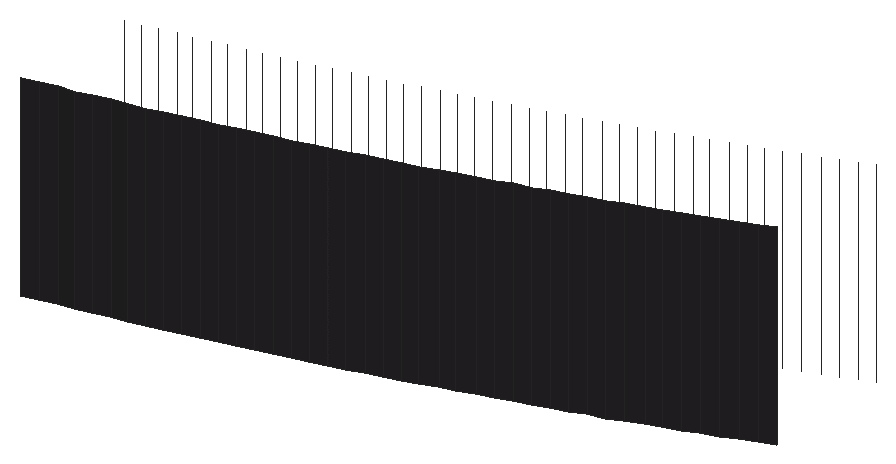
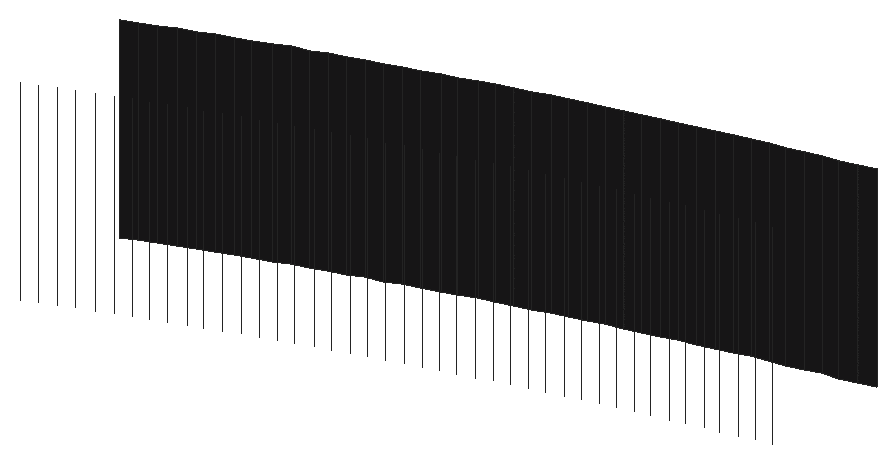
# SketchUp Ruby script. Lengths in inches.
U = 1.inch
M = Sketchup.active_model
def pt(a) = Geom::Point3d.new(a.map { |v| v * U })
def face(e, loops, mat)
  f = e.add_face(loops[0].map { |a| pt(a) })
  loops[1..].each { |l| e.add_face(l.map { |a| pt(a) }).erase! }
  f.material = f.back_material = mat if mat
  f
end
# faces: each face lists its corners as indices into pts; further lists are holes
def faces(e, pts, list, mat = nil) = list.each { |f| face(e, (f[0].is_a?(Array) ? f : [f]).map { |l| l.map { |i| pts[i] } }, mat) }
# xy, xz, yz: faces in a plane at the given z, y or x. An outline is a flat list of corners, or four numbers for a rectangle; further outlines are holes
def ring(l) = l.size == 4 ? [[l[0], l[1]], [l[2], l[1]], [l[2], l[3]], [l[0], l[3]]] : l.each_slice(2).to_a
def flat(e, list, mat, &to3) = list.each { |f| face(e, (f[0].is_a?(Array) ? f : [f]).map { |l| ring(l).map { |u, v| to3.(u, v) } }, mat) }
def xy(e, z, list, mat = nil) = flat(e, list, mat) { |x, y| [x, y, z] }
def xz(e, y, list, mat = nil) = flat(e, list, mat) { |x, z| [x, y, z] }
def yz(e, x, list, mat = nil) = flat(e, list, mat) { |y, z| [x, y, z] }
def lines(e, pts, list) = list.each { |a, b| e.add_line(pt(pts[a]), pt(pts[b])) }
# prism: a flat outline (further loops are holes) pulled along v
def prism(e, loops, v, mat = nil)
  f = face(e, loops, mat); d = Geom::Vector3d.new(v.map { |x| x * U })
  f.pushpull(f.normal.samedirection?(d) ? d.length : -d.length)
end
def box(e, o, s, mat = nil) = prism(e, [[o, [o[0] + s[0], o[1], o[2]], [o[0] + s[0], o[1] + s[1], o[2]], [o[0], o[1] + s[1], o[2]]]], [0, 0, s[2]], mat)
def at(x, y, z, deg = 0) = Geom::Transformation.translation(pt([x, y, z])) * Geom::Transformation.rotation(ORIGIN, Z_AXIS, deg.degrees)
def axes(o, x, y, z) = Geom::Transformation.new([*x, 0, *y, 0, *z, 0, *pt(o).to_a, 1])
def part(name) = M.definitions.add(name)
# library, detail: a bought-in or finely detailed component or shape, given as its bounding box
def library(name, o, s) = part(name).tap { |d| box(d.entities, o, s) }
def detail(e, o, s) = box(e.add_group.entities, o, s)
def put(e, d, t, mat = nil) = e.add_instance(d, t).tap { |i| i.material = mat if mat }
def group(e, t, mat = nil) = e.add_group.tap { |g| g.transformation = t; g.material = mat if mat }.entities
root = M.entities
M.materials.add("Marble_07_1K").color = [36, 34, 36]
p = [[350.16,772.86,18],[350.24,772.88,18],[350.24,772.88,19],[350.16,772.86,19],[350.32,772.9,18],[350.32,772.9,19],
  [350.4,772.91,18],[350.4,772.91,19],[350.47,772.93,18],[350.47,772.93,19],[350.55,772.95,18],[350.55,772.95,19],
  [350.63,772.96,18],[350.63,772.96,19],[350.71,772.98,18],[350.71,772.98,19],[350.78,773,18],[350.78,773,19],
  [350.86,773.02,18],[350.86,773.02,19],[350.9375,773.04,18],[350.9375,773.04,19],[351.02,773.06,18],[351.02,773.06,19],
  [351.09,773.08,18],[351.09,773.08,19],[351.17,773.1,18],[351.17,773.1,19],[351.25,773.12,18],[351.25,773.12,19],
  [351.33,773.14,18],[351.33,773.14,19],[351.4,773.16,18],[351.4,773.16,19],[351.48,773.18,18],[351.48,773.18,19],
  [351.56,773.2,18],[351.56,773.2,19],[351.63,773.23,18],[351.63,773.23,19],[351.71,773.25,18],[351.71,773.25,19],
  [351.79,773.27,18],[351.79,773.27,19],[351.86,773.29,18],[351.86,773.29,19],[351.9375,773.32,18],[351.9375,773.32,19],
  [352.01,773.34,18],[352.01,773.34,19],[352.09,773.37,18],[352.09,773.37,19],[352.17,773.39,18],[352.17,773.39,19],
  [352.24,773.42,18],[352.24,773.42,19],[352.32,773.44,18],[352.32,773.44,19],[352.39,773.47,18],[352.39,773.47,19],
  [352.47,773.49,18],[352.47,773.49,19],[352.54,773.52,18],[352.54,773.52,19],[352.62,773.54,18],[352.62,773.54,19],
  [352.69,773.57,18],[352.69,773.57,19],[352.77,773.6,18],[352.77,773.6,19],[352.84,773.625,18],[352.84,773.625,19],
  [352.92,773.65,18],[352.92,773.65,19],[352.99,773.68,18],[352.99,773.68,19],[353.07,773.71,18],[353.07,773.71,19],
  [353.14,773.74,18],[353.14,773.74,19],[353.22,773.77,18],[353.22,773.77,19],[353.29,773.8,18],[353.29,773.8,19],
  [350.19,773.49,18],[350.19,773.49,19],[350.27,773.5,18],[350.27,773.5,19],[350.34,773.52,18],[350.34,773.52,19],
  [350.42,773.54,18],[350.42,773.54,19],[350.49,773.55,18],[350.49,773.55,19],[350.57,773.57,18],[350.57,773.57,19],
  [350.64,773.59,18],[350.64,773.59,19],[350.72,773.61,18],[350.72,773.61,19],[350.79,773.625,18],[350.79,773.625,19],
  [350.87,773.64,18],[350.87,773.64,19],[350.94,773.66,18],[350.94,773.66,19],[351.02,773.68,18],[351.02,773.68,19],
  [351.09,773.7,18],[351.09,773.7,19],[351.17,773.72,18],[351.17,773.72,19],[351.24,773.74,18],[351.24,773.74,19],
  [351.32,773.76,18],[351.32,773.76,19],[351.39,773.78,18],[351.39,773.78,19],[351.46,773.81,18],[351.46,773.81,19],
  [351.54,773.83,18],[351.54,773.83,19],[351.61,773.85,18],[351.61,773.85,19],[351.68,773.87,18],[351.68,773.87,19],
  [351.76,773.89,18],[351.76,773.89,19],[351.83,773.92,18],[351.83,773.92,19],[351.91,773.94,18],[351.91,773.94,19],
  [351.98,773.96,18],[351.98,773.96,19],[352.05,773.99,18],[352.05,773.99,19],[352.125,774.01,18],[352.125,774.01,19],
  [352.2,774.04,18],[352.2,774.04,19],[352.27,774.0625,18],[352.27,774.0625,19],[352.34,774.09,18],[352.34,774.09,19],
  [352.42,774.11,18],[352.42,774.11,19],[352.49,774.14,18],[352.49,774.14,19],[352.5625,774.17,18],[352.5625,774.17,19],
  [352.63,774.19,18],[352.63,774.19,19],[352.71,774.22,18],[352.71,774.22,19],[352.78,774.25,18],[352.78,774.25,19],
  [352.85,774.27,18],[352.85,774.27,19],[352.92,774.3,18],[352.92,774.3,19],[352.99,774.33,18],[352.99,774.33,19],
  [353.07,774.36,18],[353.07,774.36,19],[353.14,774.39,18],[353.14,774.39,19],[353.21,774.42,18],[353.21,774.42,19],
  [353.28,774.45,18],[353.28,774.45,19]]
faces(root,p,[[0,1,2,3],[1,4,5,2],[4,6,7,5],[6,8,9,7],[8,10,11,9],[10,12,13,11],[12,14,15,13],[14,16,17,15],
  [16,18,19,17],[18,20,21,19],[20,22,23,21],[22,24,25,23],[24,26,27,25],[26,28,29,27],[28,30,31,29],[30,32,33,31],
  [32,34,35,33],[34,36,37,35],[36,38,39,37],[38,40,41,39],[40,42,43,41],[42,44,45,43],[44,46,47,45],[46,48,49,47],
  [48,50,51,49],[50,52,53,51],[52,54,55,53],[54,56,57,55],[56,58,59,57],[58,60,61,59],[60,62,63,61],[62,64,65,63],
  [64,66,67,65],[66,68,69,67],[68,70,71,69],[70,72,73,71],[72,74,75,73],[74,76,77,75],[76,78,79,77],[78,80,81,79],
  [80,82,83,81]],"Marble_07_1K")
lines(root,p,[[84,85],[86,87],[88,89],[90,91],[92,93],[94,95],[96,97],[98,99],[100,101],[102,103],[104,105],[106,107],
  [108,109],[110,111],[112,113],[114,115],[116,117],[118,119],[120,121],[122,123],[124,125],[126,127],[128,129],[130,131],
  [132,133],[134,135],[136,137],[138,139],[140,141],[142,143],[144,145],[146,147],[148,149],[150,151],[152,153],[154,155],
  [156,157],[158,159],[160,161],[162,163],[164,165],[166,167],[168,169]])
